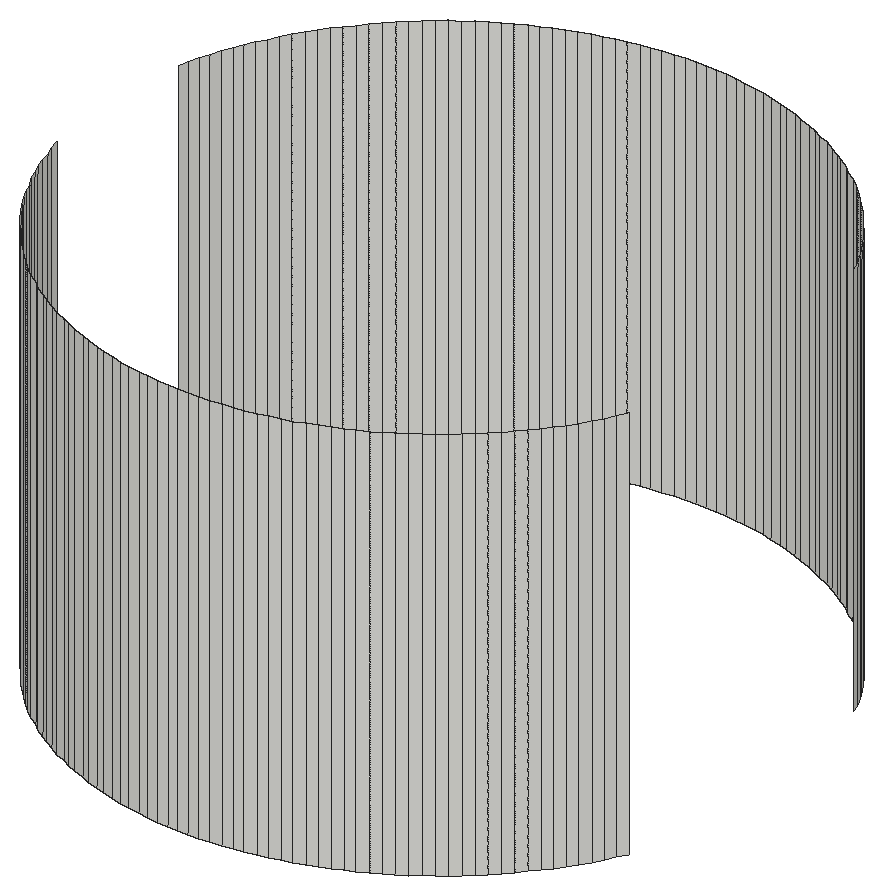
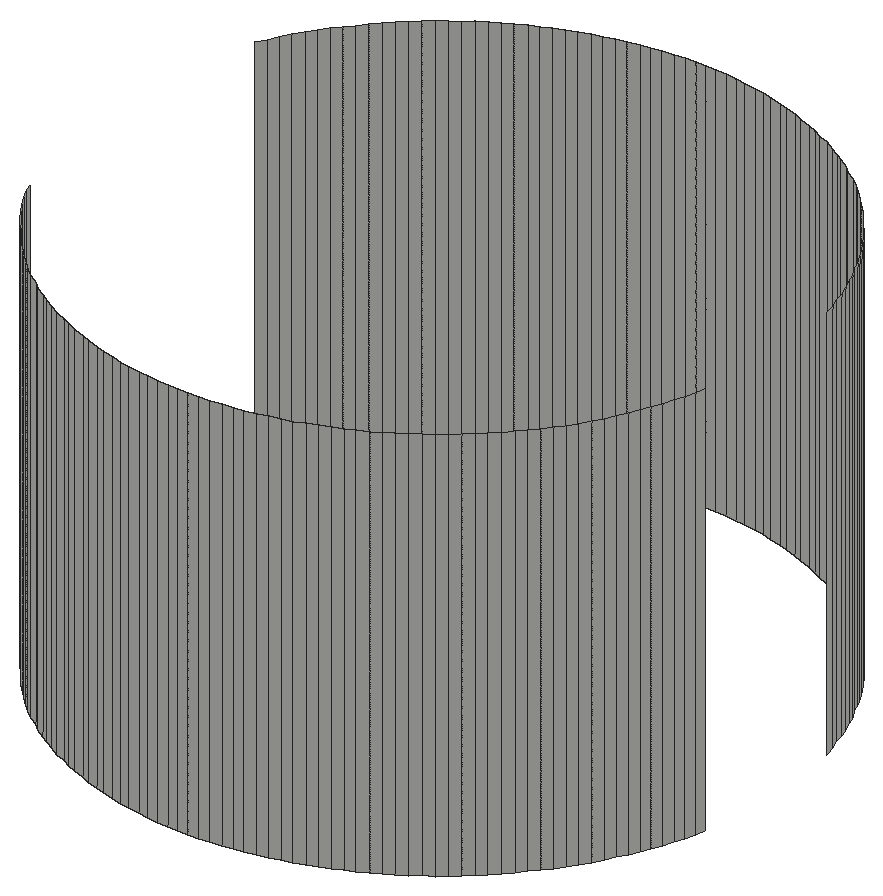
# SketchUp Ruby script. Lengths in inches.
U = 1.inch
M = Sketchup.active_model
def pt(a) = Geom::Point3d.new(a.map { |v| v * U })
def face(e, loops, mat)
  f = e.add_face(loops[0].map { |a| pt(a) })
  loops[1..].each { |l| e.add_face(l.map { |a| pt(a) }).erase! }
  f.material = f.back_material = mat if mat
  f
end
# faces: each face lists its corners as indices into pts; further lists are holes
def faces(e, pts, list, mat = nil) = list.each { |f| face(e, (f[0].is_a?(Array) ? f : [f]).map { |l| l.map { |i| pts[i] } }, mat) }
# xy, xz, yz: faces in a plane at the given z, y or x. An outline is a flat list of corners, or four numbers for a rectangle; further outlines are holes
def ring(l) = l.size == 4 ? [[l[0], l[1]], [l[2], l[1]], [l[2], l[3]], [l[0], l[3]]] : l.each_slice(2).to_a
def flat(e, list, mat, &to3) = list.each { |f| face(e, (f[0].is_a?(Array) ? f : [f]).map { |l| ring(l).map { |u, v| to3.(u, v) } }, mat) }
def xy(e, z, list, mat = nil) = flat(e, list, mat) { |x, y| [x, y, z] }
def xz(e, y, list, mat = nil) = flat(e, list, mat) { |x, z| [x, y, z] }
def yz(e, x, list, mat = nil) = flat(e, list, mat) { |y, z| [x, y, z] }
def lines(e, pts, list) = list.each { |a, b| e.add_line(pt(pts[a]), pt(pts[b])) }
# prism: a flat outline (further loops are holes) pulled along v
def prism(e, loops, v, mat = nil)
  f = face(e, loops, mat); d = Geom::Vector3d.new(v.map { |x| x * U })
  f.pushpull(f.normal.samedirection?(d) ? d.length : -d.length)
end
def box(e, o, s, mat = nil) = prism(e, [[o, [o[0] + s[0], o[1], o[2]], [o[0] + s[0], o[1] + s[1], o[2]], [o[0], o[1] + s[1], o[2]]]], [0, 0, s[2]], mat)
def at(x, y, z, deg = 0) = Geom::Transformation.translation(pt([x, y, z])) * Geom::Transformation.rotation(ORIGIN, Z_AXIS, deg.degrees)
def axes(o, x, y, z) = Geom::Transformation.new([*x, 0, *y, 0, *z, 0, *pt(o).to_a, 1])
def part(name) = M.definitions.add(name)
# library, detail: a bought-in or finely detailed component or shape, given as its bounding box
def library(name, o, s) = part(name).tap { |d| box(d.entities, o, s) }
def detail(e, o, s) = box(e.add_group.entities, o, s)
def put(e, d, t, mat = nil) = e.add_instance(d, t).tap { |i| i.material = mat if mat }
def group(e, t, mat = nil) = e.add_group.tap { |g| g.transformation = t; g.material = mat if mat }.entities
root = M.entities
xz(root,124,[[186.97,366,187.05,369],[187.05,366,187.125,369],[187.125,366,187.2,369],[187.2,366,187.28,369]])
xz(root,129,[[186.97,366,187.05,369],[187.05,366,187.125,369],[187.125,366,187.2,369],[187.2,366,187.28,369]])
p = [[186.66,124.04,366],[186.58,124.06,366],[186.58,124.06,369],[186.66,124.04,369],[186.73,124.03,366],[186.73,124.03,369],
  [186.8125,124.02,366],[186.8125,124.02,369],[186.89,124.01,366],[186.89,124.01,369],[186.97,124,366],[186.97,124,369],
  [187.36,124.01,366],[187.28,124,366],[187.28,124,369],[187.36,124.01,369],[187.4375,124.02,366],[187.4375,124.02,369],
  [187.52,124.03,366],[187.52,124.03,369],[187.59,124.04,366],[187.59,124.04,369],[187.67,124.06,366],[187.67,124.06,369],
  [186.28,124.15,366],[186.2,124.18,366],[186.2,124.18,369],[186.28,124.15,369],[186.35,124.12,366],[186.35,124.12,369],
  [186.43,124.1,366],[186.43,124.1,369],[186.5,124.08,366],[186.5,124.08,369],[187.75,124.08,366],[187.75,124.08,369],
  [187.82,124.1,366],[187.82,124.1,369],[187.9,124.12,366],[187.9,124.12,369],[187.97,124.15,366],[187.97,124.15,369],
  [188.05,124.18,366],[188.05,124.18,369],[186.0625,124.24,366],[185.99,124.27,366],[185.99,124.27,369],[186.0625,124.24,369],
  [186.13,124.21,366],[186.13,124.21,369],[188.12,124.21,366],[188.12,124.21,369],[188.1875,124.24,366],[188.1875,124.24,369],
  [188.26,124.27,366],[188.26,124.27,369],[185.85,124.35,366],[185.79,124.39,366],[185.79,124.39,369],[185.85,124.35,369],
  [185.92,124.31,366],[185.92,124.31,369],[188.33,124.31,366],[188.33,124.31,369],[188.4,124.35,366],[188.4,124.35,369],
  [188.46,124.39,366],[188.46,124.39,369],[185.72,124.43,366],[185.66,124.48,366],[185.66,124.48,369],[185.72,124.43,369],
  [188.53,124.43,366],[188.53,124.43,369],[188.59,124.48,366],[188.59,124.48,369],[185.59,124.52,366],[185.53,124.57,366],
  [185.53,124.57,369],[185.59,124.52,369],[188.66,124.52,366],[188.66,124.52,369],[188.72,124.57,366],[188.72,124.57,369],
  [185.47,124.625,366],[185.41,124.68,366],[185.41,124.68,369],[185.47,124.625,369],[188.78,124.625,366],[188.78,124.625,369],
  [188.84,124.68,366],[188.84,124.68,369],[185.36,124.73,366],[185.3,124.79,366],[185.3,124.79,369],[185.36,124.73,369],
  [188.89,124.73,366],[188.89,124.73,369],[188.95,124.79,366],[188.95,124.79,369],[185.25,124.85,366],[185.2,124.91,366],
  [185.2,124.91,369],[185.25,124.85,369],[189,124.85,366],[189,124.85,369],[189.05,124.91,366],[189.05,124.91,369],
  [185.15,124.97,366],[185.15,124.97,369],[189.1,124.97,366],[189.1,124.97,369],[185.1,125.03,366],[185.06,125.09,366],
  [185.06,125.09,369],[185.1,125.03,369],[189.15,125.03,366],[189.15,125.03,369],[189.19,125.09,366],[189.19,125.09,369],
  [185.01,125.16,366],[185.01,125.16,369],[189.24,125.16,366],[189.24,125.16,369],[184.97,125.23,366],[184.93,125.3,366],
  [184.93,125.3,369],[184.97,125.23,369],[189.28,125.23,366],[189.28,125.23,369],[189.32,125.3,366],[189.32,125.3,369],
  [184.9,125.37,366],[184.9,125.37,369],[189.35,125.37,366],[189.35,125.37,369],[184.86,125.4375,366],[184.83,125.51,366],
  [184.83,125.51,369],[184.86,125.4375,369],[189.39,125.4375,366],[189.39,125.4375,369],[184.8,125.58,366],[184.8,125.58,369],
  [184.77,125.65,366],[184.77,125.65,369],[184.75,125.73,366],[184.72,125.8,366],[184.72,125.8,369],[184.75,125.73,369],
  [184.7,125.88,366],[184.7,125.88,369],[184.69,127.05,366],[184.7,127.12,366],[184.7,127.12,369],[184.69,127.05,369],
  [184.72,127.2,366],[184.72,127.2,369],[184.75,127.27,366],[184.75,127.27,369],[184.77,127.35,366],[184.77,127.35,369],
  [184.8,127.42,366],[184.8,127.42,369],[184.83,127.49,366],[184.83,127.49,369],[184.86,127.5625,366],[184.86,127.5625,369],
  [184.9,127.63,366],[184.9,127.63,369],[184.93,127.7,366],[184.93,127.7,369],[189.32,127.7,366],[189.35,127.63,366],
  [189.35,127.63,369],[189.32,127.7,369],[184.97,127.77,366],[184.97,127.77,369],[189.28,127.77,366],[189.28,127.77,369],
  [185.01,127.84,366],[185.01,127.84,369],[185.06,127.91,366],[185.06,127.91,369],[189.19,127.91,366],[189.24,127.84,366],
  [189.24,127.84,369],[189.19,127.91,369],[185.1,127.97,366],[185.1,127.97,369],[189.15,127.97,366],[189.15,127.97,369],
  [185.15,128.03,366],[185.15,128.03,369],[185.2,128.09,366],[185.2,128.09,369],[189.05,128.09,366],[189.1,128.03,366],
  [189.1,128.03,369],[189.05,128.09,369],[185.25,128.15,366],[185.25,128.15,369],[189,128.15,366],[189,128.15,369],
  [185.3,128.21,366],[185.3,128.21,369],[185.36,128.27,366],[185.36,128.27,369],[188.89,128.27,366],[188.95,128.21,366],
  [188.95,128.21,369],[188.89,128.27,369],[185.41,128.32,366],[185.41,128.32,369],[185.47,128.375,366],[185.47,128.375,369],
  [188.78,128.375,366],[188.84,128.32,366],[188.84,128.32,369],[188.78,128.375,369],[185.53,128.43,366],[185.53,128.43,369],
  [185.59,128.48,366],[185.59,128.48,369],[188.66,128.48,366],[188.72,128.43,366],[188.72,128.43,369],[188.66,128.48,369],
  [185.66,128.52,366],[185.66,128.52,369],[185.72,128.57,366],[185.72,128.57,369],[188.53,128.57,366],[188.59,128.52,366],
  [188.59,128.52,369],[188.53,128.57,369],[185.79,128.61,366],[185.79,128.61,369],[185.85,128.65,366],[185.85,128.65,369],
  [188.4,128.65,366],[188.46,128.61,366],[188.46,128.61,369],[188.4,128.65,369],[185.92,128.69,366],[185.92,128.69,369],
  [185.99,128.73,366],[185.99,128.73,369],[186.0625,128.76,366],[186.0625,128.76,369],[188.1875,128.76,366],[188.26,128.73,366],
  [188.26,128.73,369],[188.1875,128.76,369],[188.33,128.69,366],[188.33,128.69,369],[186.13,128.79,366],[186.13,128.79,369],
  [186.2,128.82,366],[186.2,128.82,369],[186.28,128.85,366],[186.28,128.85,369],[187.97,128.85,366],[188.05,128.82,366],
  [188.05,128.82,369],[187.97,128.85,369],[188.12,128.79,366],[188.12,128.79,369],[186.35,128.88,366],[186.35,128.88,369],
  [186.43,128.9,366],[186.43,128.9,369],[186.5,128.92,366],[186.5,128.92,369],[186.58,128.94,366],[186.58,128.94,369],
  [186.66,128.96,366],[186.66,128.96,369],[187.59,128.96,366],[187.67,128.94,366],[187.67,128.94,369],[187.59,128.96,369],
  [187.75,128.92,366],[187.75,128.92,369],[187.82,128.9,366],[187.82,128.9,369],[187.9,128.88,366],[187.9,128.88,369],
  [186.73,128.97,366],[186.73,128.97,369],[186.8125,128.98,366],[186.8125,128.98,369],[186.89,128.99,366],[186.89,128.99,369],
  [186.97,129,366],[186.97,129,369],[187.28,129,366],[187.36,128.99,366],[187.36,128.99,369],[187.28,129,369],
  [187.4375,128.98,366],[187.4375,128.98,369],[187.52,128.97,366],[187.52,128.97,369]]
faces(root,p,[[0,1,2,3],[4,0,3,5],[6,4,5,7],[8,6,7,9],[10,8,9,11],[12,13,14,15],[16,12,15,17],[18,16,17,19],
  [20,18,19,21],[22,20,21,23],[24,25,26,27],[28,24,27,29],[30,28,29,31],[32,30,31,33],[1,32,33,2],[34,22,23,35],
  [36,34,35,37],[38,36,37,39],[40,38,39,41],[42,40,41,43],[44,45,46,47],[48,44,47,49],[25,48,49,26],[50,42,43,51],
  [52,50,51,53],[54,52,53,55],[56,57,58,59],[60,56,59,61],[45,60,61,46],[62,54,55,63],[64,62,63,65],[66,64,65,67],
  [68,69,70,71],[57,68,71,58],[72,66,67,73],[74,72,73,75],[76,77,78,79],[69,76,79,70],[80,74,75,81],[82,80,81,83],
  [84,85,86,87],[77,84,87,78],[88,82,83,89],[90,88,89,91],[92,93,94,95],[85,92,95,86],[96,90,91,97],[98,96,97,99],
  [100,101,102,103],[93,100,103,94],[104,98,99,105],[106,104,105,107],[101,108,109,102],[110,106,107,111],[112,113,114,115],[108,112,115,109],
  [116,110,111,117],[118,116,117,119],[113,120,121,114],[122,118,119,123],[124,125,126,127],[120,124,127,121],[128,122,123,129],[130,128,129,131],
  [125,132,133,126],[134,130,131,135],[136,137,138,139],[132,136,139,133],[140,134,135,141],[137,142,143,138],[142,144,145,143],[146,147,148,149],
  [144,146,149,145],[147,150,151,148],[152,153,154,155],[153,156,157,154],[156,158,159,157],[158,160,161,159],[160,162,163,161],[162,164,165,163],
  [164,166,167,165],[166,168,169,167],[168,170,171,169],[172,173,174,175],[170,176,177,171],[178,172,175,179],[176,180,181,177],[180,182,183,181],
  [184,185,186,187],[185,178,179,186],[182,188,189,183],[190,184,187,191],[188,192,193,189],[192,194,195,193],[196,197,198,199],[197,190,191,198],
  [194,200,201,195],[202,196,199,203],[200,204,205,201],[204,206,207,205],[208,209,210,211],[209,202,203,210],[206,212,213,207],[212,214,215,213],
  [216,217,218,219],[217,208,211,218],[214,220,221,215],[220,222,223,221],[224,225,226,227],[225,216,219,226],[222,228,229,223],[228,230,231,229],
  [232,233,234,235],[233,224,227,234],[230,236,237,231],[236,238,239,237],[240,241,242,243],[241,232,235,242],[238,244,245,239],[244,246,247,245],
  [246,248,249,247],[250,251,252,253],[251,254,255,252],[254,240,243,255],[248,256,257,249],[256,258,259,257],[258,260,261,259],[262,263,264,265],
  [263,266,267,264],[266,250,253,267],[260,268,269,261],[268,270,271,269],[270,272,273,271],[272,274,275,273],[274,276,277,275],[278,279,280,281],
  [279,282,283,280],[282,284,285,283],[284,286,287,285],[286,262,265,287],[276,288,289,277],[288,290,291,289],[290,292,293,291],[292,294,295,293],
  [296,297,298,299],[297,300,301,298],[300,302,303,301],[302,278,281,303]])
